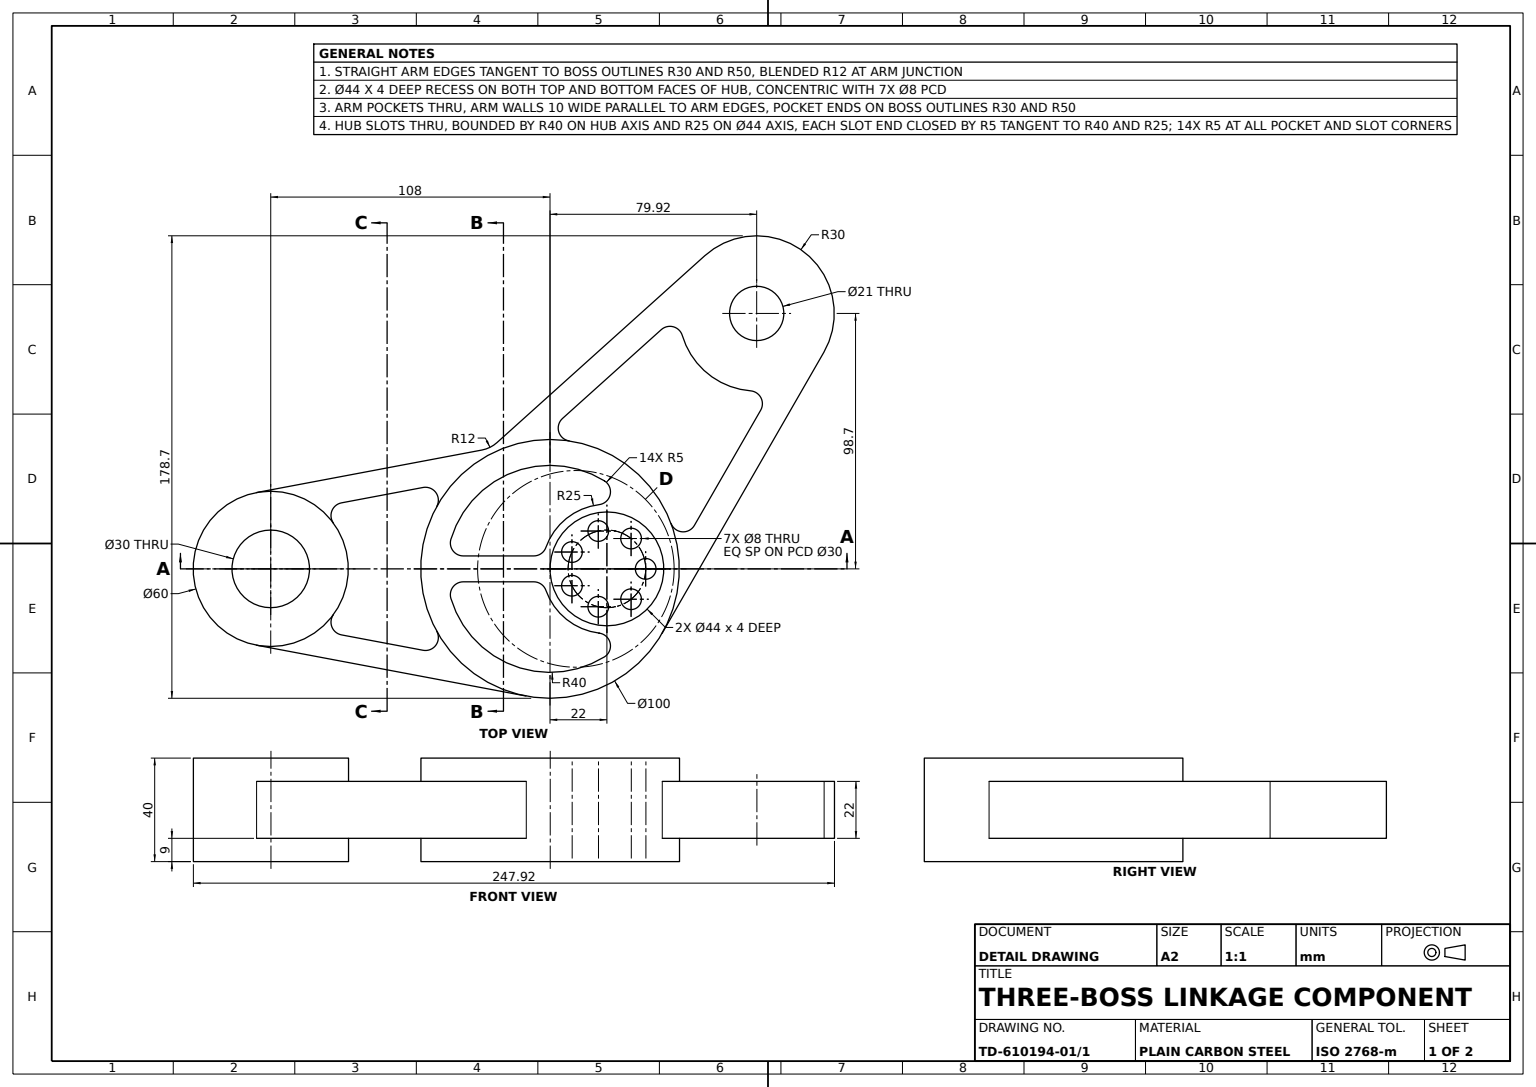
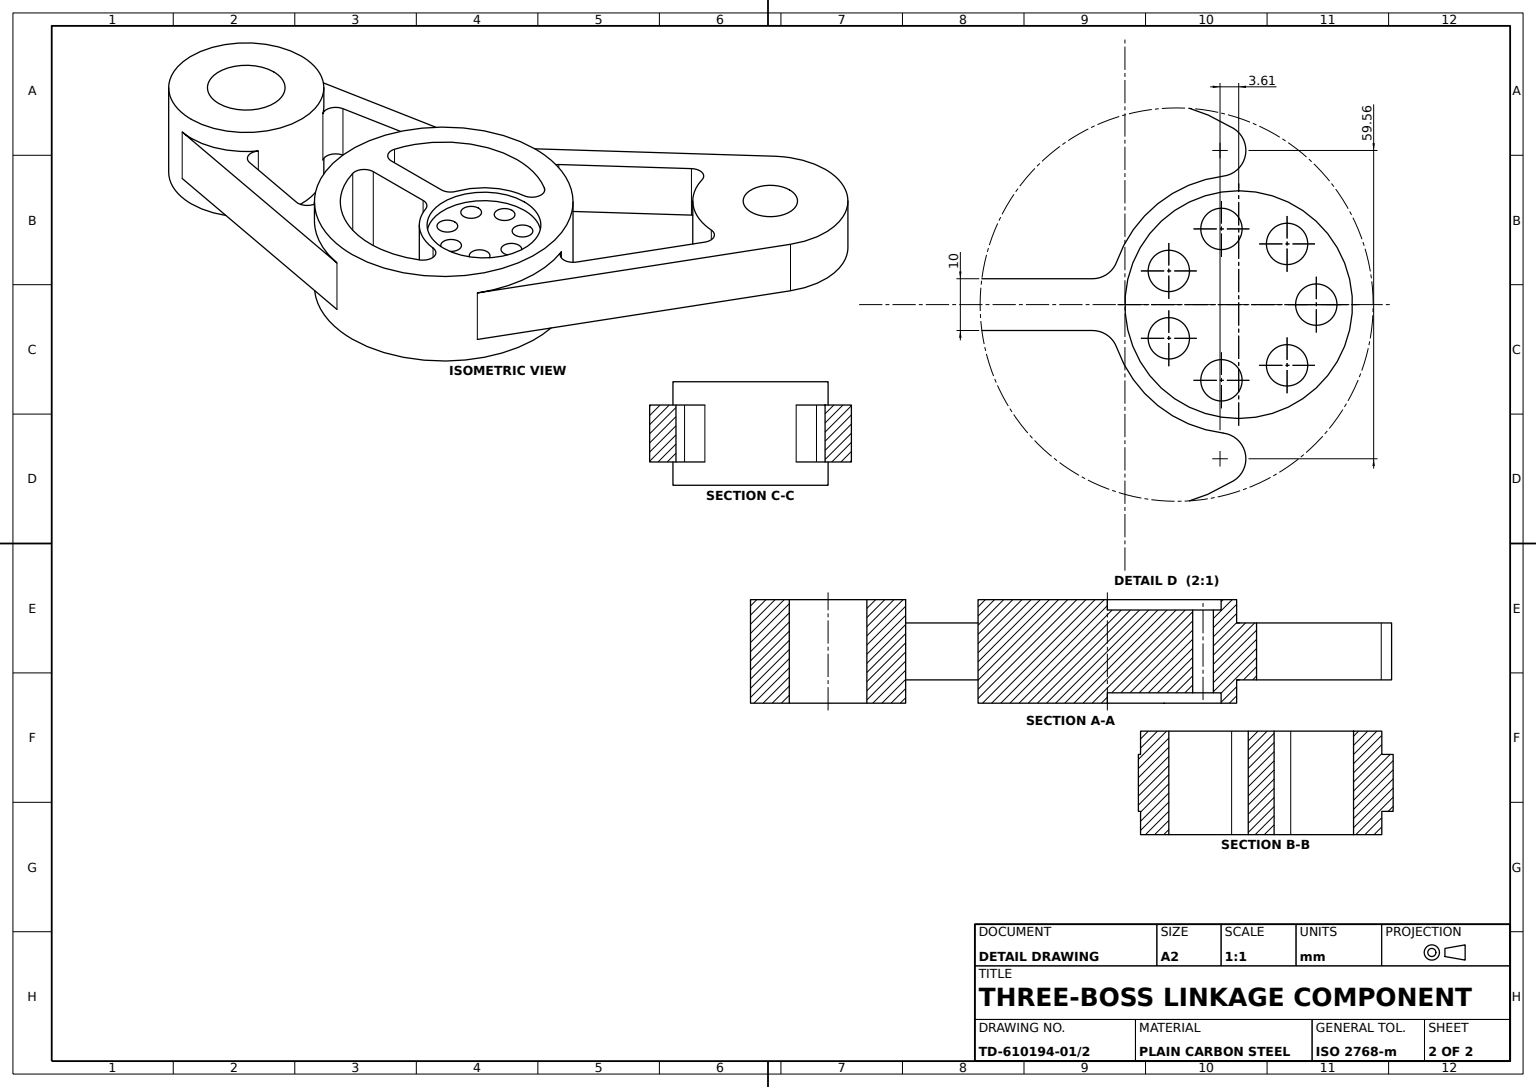
solid
v1 (46.8215331881,11,-17.5426346343)
v2 (46.8215331881,-11,-17.5426346343)
e1 v1 v2 LINE
v3 (55.8364585363,11,-16.8014849975)
e2 v1 v3 CIRCLE(AX(P(51.5036865069,11,-19.2968980978),D(0,1,0),D(0,0,-1)),5)
v4 (55.8364585363,-11,-16.8014849975)
e3 v3 v4 LINE
e4 v2 v4 CIRCLE(AX(P(51.5036865069,-11,-19.2968980978),D(0,1,0),D(0,0,-1)),5)
face CYL(AX(P(51.5036865069,11,-19.2968980978),D(0,-1,0),D(0,0,-1)),5) rev [-e1 e2 e3 -e4]
v5 (22,16,-22)
v6 (22,20,-22)
e5 v5 v6 LINE
v7 (22,16,22)
e6 v7 v5 CIRCLE(AX(P(22,16,0),D(0,1,0),D(0,0,1)),22)
v8 (22,20,22)
e7 v7 v8 LINE
e8 v8 v6 CIRCLE(AX(P(22,20,0),D(0,1,0),D(0,0,1)),22)
face CYL(AX(P(22,16,0),D(0,1,0),D(0,0,1)),22) rev [-e5 -e6 e7 e8]
v9 (-48.1740660132,11,-31.5378854424)
v10 (-43.7946054666,11,-24.1253504021)
e9 v9 v10 CIRCLE(AX(P(-48.1740660132,11,-26.5378854424),D(0,-1,0),D(0,0,1)),5)
v11 (-48.1740660132,-11,-31.5378854424)
e10 v9 v11 LINE
v12 (-43.7946054666,-11,-24.1253504021)
e11 v11 v12 CIRCLE(AX(P(-48.1740660132,-11,-26.5378854424),D(0,-1,0),D(0,0,1)),5)
e12 v10 v12 LINE
face CYL(AX(P(-48.1740660132,11,-26.5378854424),D(0,-1,0),D(0,0,-1)),5) rev [-e9 e10 e11 -e12]
v13 (-80.6278859801,11,25.5101425728)
v14 (-80.6278859801,-11,25.5101425728)
e13 v13 v14 LINE
v15 (-83.7445371893,-11,17.6542494556)
e14 v15 v14 CIRCLE(AX(P(-79.7019600542,-11,20.5966243649),D(0,1,0),D(0,0,-1)),5)
v16 (-83.7445371893,11,17.6542494556)
e15 v16 v15 LINE
e16 v16 v13 CIRCLE(AX(P(-79.7019600542,11,20.5966243649),D(0,1,0),D(0,0,-1)),5)
face CYL(AX(P(-79.7019600542,11,20.5966243649),D(0,-1,0),D(0,0,-1)),5) rev [e13 -e14 -e15 e16]
v17 (18.9886363636,-20,-24.8179710905)
v18 (21.012987013,-20,-34.0360746384)
e17 v17 v18 CIRCLE(AX(P(18.3863636364,-20,-29.7815653086),D(0,1,0),D(0,0,-1)),5)
v19 (18.9886363636,20,-24.8179710905)
e18 v19 v17 LINE
v20 (21.012987013,20,-34.0360746384)
e19 v19 v20 CIRCLE(AX(P(18.3863636364,20,-29.7815653086),D(0,1,0),D(0,0,-1)),5)
e20 v20 v18 LINE
face CYL(AX(P(18.3863636364,11,-29.7815653086),D(0,-1,0),D(0,0,-1)),5) rev [-e17 -e18 e19 e20]
v21 (21.012987013,20,34.0360746384)
v22 (21.012987013,-20,34.0360746384)
e21 v21 v22 LINE
v23 (-38.3325939,-20,11.4285714286)
e22 v23 v22 CIRCLE(AX(P(0,-20,0),D(0,1,0),D(0,0,1)),40)
v24 (-38.3325939,20,11.4285714286)
e23 v24 v23 LINE
e24 v24 v21 CIRCLE(AX(P(0,20,0),D(0,1,0),D(0,0,1)),40)
face CYL(AX(P(0,11,0),D(0,-1,0),D(0,0,-1)),40) rev [e21 -e22 -e23 e24]
v25 (-108,-11,30)
v26 (-108,-20,30)
e25 v25 v26 LINE
v27 (-108,-20,-30)
e26 v26 v27 CIRCLE(AX(P(-108,-20,0),D(0,1,0),D(0,0,1)),30)
v28 (-108,-11,-30)
e27 v28 v27 LINE
v29 (-83.7445371893,-11,-17.6542494556)
e28 v28 v29 CIRCLE(AX(P(-108,-11,0),D(0,-1,0),D(0,0,1)),30)
v30 (-83.7445371893,11,-17.6542494556)
e29 v30 v29 LINE
v31 (-108,11,-30)
e30 v31 v30 CIRCLE(AX(P(-108,11,0),D(0,-1,0),D(0,0,1)),30)
v32 (-108,20,-30)
e31 v32 v31 LINE
v33 (-108,20,30)
e32 v33 v32 CIRCLE(AX(P(-108,20,0),D(0,1,0),D(0,0,1)),30)
v34 (-108,11,30)
e33 v33 v34 LINE
e34 v34 v16 CIRCLE(AX(P(-108,11,0),D(0,1,0),D(0,0,1)),30)
e35 v25 v15 CIRCLE(AX(P(-108,-11,0),D(0,1,0),D(0,0,1)),30)
face CYL(AX(P(-108,20,0),D(0,-1,0),D(0,0,-1)),30) [e25 e26 -e27 e28 -e29 -e30 -e31 -e32 e33 e34 e15 -e35]
v35 (-38.3325939,20,-11.4285714286)
v36 (-38.3325939,-20,-11.4285714286)
e36 v35 v36 LINE
v37 (0,-20,-40)
e37 v37 v36 CIRCLE(AX(P(0,-20,0),D(0,1,0),D(0,0,1)),40)
v38 (0,20,-40)
e38 v38 v37 LINE
e39 v38 v35 CIRCLE(AX(P(0,20,0),D(0,1,0),D(0,0,1)),40)
face CYL(AX(P(0,11,0),D(0,-1,0),D(0,0,-1)),40) rev [e36 -e37 -e38 e39]
v39 (-49.0999919392,-11,-31.4514036503)
e40 v39 v11 CIRCLE(AX(P(-48.1740660132,-11,-26.5378854424),D(0,-1,0),D(0,0,1)),5)
v40 (-49.0999919392,11,-31.4514036503)
e41 v40 v9 CIRCLE(AX(P(-48.1740660132,11,-26.5378854424),D(0,-1,0),D(0,0,1)),5)
e42 v40 v39 LINE
face CYL(AX(P(-48.1740660132,11,-26.5378854424),D(0,-1,0),D(0,0,-1)),5) rev [e40 -e10 -e41 e42]
v41 (81.472399581,11,-61.3130283134)
v42 (81.472399581,-11,-61.3130283134)
e43 v41 v42 LINE
e44 v4 v42 LINE
e45 v3 v41 LINE
face PLANE(AX(P(55.8364585363,11,-16.8014849975),D(-0.8665544059,0,-0.4990826201),D(-0.4990826201,0,0.8665544059))) [e43 -e44 -e3 e45]
v43 (-33.5410196625,-20,5)
e46 v43 v23 CIRCLE(AX(P(-33.5410196625,-20,10),D(0,1,0),D(0,0,1)),5)
v44 (18.9886363636,-20,24.8179710905)
e47 v22 v44 CIRCLE(AX(P(18.3863636364,-20,29.7815653086),D(0,1,0),D(0,0,1)),5)
v45 (-1.5702260396,-20,8.3333333333)
e48 v44 v45 CIRCLE(AX(P(22,-20,0),D(0,-1,0),D(0,0,1)),25)
v46 (-6.2842712475,-20,5)
e49 v45 v46 CIRCLE(AX(P(-6.2842712475,-20,10),D(0,1,0),D(0,0,-1)),5)
e50 v46 v43 LINE
v47 (-33.5410196625,-20,-5)
e51 v36 v47 CIRCLE(AX(P(-33.5410196625,-20,-10),D(0,1,0),D(0,0,-1)),5)
v48 (-6.2842712475,-20,-5)
e52 v47 v48 LINE
v49 (-1.5702260396,-20,-8.3333333333)
e53 v48 v49 CIRCLE(AX(P(-6.2842712475,-20,-10),D(0,1,0),D(0,0,-1)),5)
e54 v49 v17 CIRCLE(AX(P(22,-20,0),D(0,-1,0),D(0,0,1)),25)
e55 v18 v37 CIRCLE(AX(P(0,-20,0),D(0,1,0),D(0,0,1)),40)
v50 (22,-20,22)
v51 (22,-20,-22)
e56 v50 v51 CIRCLE(AX(P(22,-20,0),D(0,1,0),D(0,0,1)),22)
e57 v51 v50 CIRCLE(AX(P(22,-20,0),D(0,1,0),D(0,0,1)),22)
v52 (0,-20,-50)
v53 (0,-20,50)
e58 v52 v53 CIRCLE(AX(P(0,-20,0),D(0,1,0),D(0,0,1)),50)
e59 v53 v52 CIRCLE(AX(P(0,-20,0),D(0,1,0),D(0,0,1)),50)
face PLANE(AX(P(0,-20,0),D(0,1,0),D(0,0,1))) rev [e46 e22 e47 e48 e49 e50] [e51 e52 e53 e54 e17 e55 e37] [e56 e57] [-e58 -e59]
v54 (-108,20,15)
v55 (-108,-20,15)
e60 v54 v55 LINE
v56 (-108,20,-15)
e61 v54 v56 CIRCLE(AX(P(-108,20,0),D(0,1,0),D(0,0,1)),15)
v57 (-108,-20,-15)
e62 v56 v57 LINE
e63 v55 v57 CIRCLE(AX(P(-108,-20,0),D(0,1,0),D(0,0,1)),15)
face CYL(AX(P(-108,20,0),D(0,-1,0),D(0,0,-1)),15) rev [-e60 e61 e62 -e63]
v58 (-33.5410196625,20,-5)
v59 (-6.2842712475,20,-5)
e64 v58 v59 LINE
e65 v59 v48 LINE
e66 v58 v47 LINE
face PLANE(AX(P(-33.5410196625,11,-5),D(0,0,-1),D(-1,0,0))) [e64 e65 -e52 -e66]
v60 (-33.5410196625,20,5)
e67 v60 v43 LINE
v61 (-6.2842712475,20,5)
e68 v61 v46 LINE
e69 v61 v60 LINE
face PLANE(AX(P(-6.2842712475,11,5),D(0,0,1),D(1,0,0))) [e67 -e50 -e68 e69]
v62 (18.6621859907,-16,-10.6239186827)
v63 (18.6621859907,-16,-18.6239186827)
e70 v62 v63 CIRCLE(AX(P(18.6621859907,-16,-14.6239186827),D(0,-1,0),D(0,0,-1)),4)
v64 (18.6621859907,16,-18.6239186827)
e71 v64 v63 LINE
v65 (18.6621859907,16,-10.6239186827)
e72 v64 v65 CIRCLE(AX(P(18.6621859907,16,-14.6239186827),D(0,1,0),D(0,0,1)),4)
e73 v65 v62 LINE
face CYL(AX(P(18.6621859907,20,-14.6239186827),D(0,-1,0),D(0,0,-1)),4) rev [e70 -e71 e72 e73]
e74 v35 v58 CIRCLE(AX(P(-33.5410196625,20,-10),D(0,1,0),D(0,0,-1)),5)
face CYL(AX(P(-33.5410196625,11,-10),D(0,-1,0),D(0,0,-1)),5) rev [e66 -e51 -e36 e74]
v66 (79.9236896633,11,-128.697537105)
v67 (79.9236896633,-11,-128.697537105)
e75 v66 v67 LINE
v68 (105.9203218398,11,-83.7250585032)
e76 v68 v66 CIRCLE(AX(P(79.9236896633,11,-98.697537105),D(0,1,0),D(0,0,1)),30)
v69 (105.9203218398,-11,-83.7250585032)
e77 v68 v69 LINE
e78 v69 v67 CIRCLE(AX(P(79.9236896633,-11,-98.697537105),D(0,1,0),D(0,0,1)),30)
face CYL(AX(P(79.9236896633,11,-98.697537105),D(0,-1,0),D(0,0,-1)),30) [-e75 -e76 e77 e78]
v70 (18.9886363636,20,24.8179710905)
e79 v70 v44 LINE
e80 v21 v70 CIRCLE(AX(P(18.3863636364,20,29.7815653086),D(0,1,0),D(0,0,1)),5)
face CYL(AX(P(18.3863636364,11,29.7815653086),D(0,-1,0),D(0,0,-1)),5) rev [e79 -e47 -e21 e80]
e81 v63 v62 CIRCLE(AX(P(18.6621859907,-16,-14.6239186827),D(0,-1,0),D(0,0,-1)),4)
e82 v65 v64 CIRCLE(AX(P(18.6621859907,16,-14.6239186827),D(0,1,0),D(0,0,1)),4)
face CYL(AX(P(18.6621859907,20,-14.6239186827),D(0,-1,0),D(0,0,-1)),4) rev [e71 e81 -e73 e82]
v71 (37,16,-4)
v72 (37,-16,-4)
e83 v71 v72 LINE
v73 (37,-16,4)
e84 v72 v73 CIRCLE(AX(P(37,-16,0),D(0,-1,0),D(0,0,-1)),4)
v74 (37,16,4)
e85 v74 v73 LINE
e86 v74 v71 CIRCLE(AX(P(37,16,0),D(0,1,0),D(0,0,1)),4)
face CYL(AX(P(37,20,0),D(0,-1,0),D(0,0,-1)),4) rev [e83 e84 -e85 e86]
v75 (59.8733918905,11,-121.0131271537)
v76 (59.8733918905,-11,-121.0131271537)
e87 v75 v76 LINE
v77 (-20.5112949272,-11,-48.7884222029)
e88 v76 v77 LINE
v78 (-20.5112949272,11,-48.7884222029)
e89 v78 v77 LINE
e90 v75 v78 LINE
face PLANE(AX(P(-20.5112949272,11,-48.7884222029),D(0.6683432591,0,0.7438530016),D(0.7438530016,0,-0.6683432591))) rev [e87 e88 -e89 -e90]
e91 v73 v72 CIRCLE(AX(P(37,-16,0),D(0,-1,0),D(0,0,-1)),4)
v79 (18.6621859907,-16,10.6239186827)
v80 (18.6621859907,-16,18.6239186827)
e92 v79 v80 CIRCLE(AX(P(18.6621859907,-16,14.6239186827),D(0,-1,0),D(0,0,-1)),4)
e93 v80 v79 CIRCLE(AX(P(18.6621859907,-16,14.6239186827),D(0,-1,0),D(0,0,-1)),4)
v81 (8.4854669815,-16,-2.5082560868)
v82 (8.4854669815,-16,-10.5082560868)
e94 v81 v82 CIRCLE(AX(P(8.4854669815,-16,-6.5082560868),D(0,-1,0),D(0,0,-1)),4)
e95 v82 v81 CIRCLE(AX(P(8.4854669815,-16,-6.5082560868),D(0,-1,0),D(0,0,-1)),4)
v83 (31.3523470279,-16,15.727472237)
v84 (31.3523470279,-16,7.727472237)
e96 v83 v84 CIRCLE(AX(P(31.3523470279,-16,11.727472237),D(0,-1,0),D(0,0,-1)),4)
e97 v84 v83 CIRCLE(AX(P(31.3523470279,-16,11.727472237),D(0,-1,0),D(0,0,-1)),4)
v85 (22,-16,-22)
v86 (22,-16,22)
e98 v85 v86 CIRCLE(AX(P(22,-16,0),D(0,1,0),D(0,0,1)),22)
e99 v86 v85 CIRCLE(AX(P(22,-16,0),D(0,1,0),D(0,0,1)),22)
v87 (8.4854669815,-16,2.5082560868)
v88 (8.4854669815,-16,10.5082560868)
e100 v87 v88 CIRCLE(AX(P(8.4854669815,-16,6.5082560868),D(0,-1,0),D(0,0,-1)),4)
e101 v88 v87 CIRCLE(AX(P(8.4854669815,-16,6.5082560868),D(0,-1,0),D(0,0,-1)),4)
v89 (31.3523470279,-16,-7.727472237)
v90 (31.3523470279,-16,-15.727472237)
e102 v89 v90 CIRCLE(AX(P(31.3523470279,-16,-11.727472237),D(0,-1,0),D(0,0,-1)),4)
e103 v90 v89 CIRCLE(AX(P(31.3523470279,-16,-11.727472237),D(0,-1,0),D(0,0,-1)),4)
face PLANE(AX(P(22,-16,0),D(0,-1,0),D(0,0,1))) [-e70 -e81] [-e91 -e84] [-e92 -e93] [-e94 -e95] [-e96 -e97] [-e98 -e99] [-e100 -e101] [-e102 -e103]
v91 (-113.5555555556,-11,29.4811092476)
e104 v91 v25 CIRCLE(AX(P(-108,-11,0),D(0,1,0),D(0,0,1)),30)
v92 (-49.0999919392,-11,31.4514036503)
e105 v14 v92 LINE
v93 (-43.7946054666,-11,24.1253504021)
e106 v92 v93 CIRCLE(AX(P(-48.1740660132,-11,26.5378854424),D(0,1,0),D(0,0,1)),5)
v94 (-9.2592592593,-11,49.1351820793)
e107 v94 v93 CIRCLE(AX(P(0,-11,0),D(0,-1,0),D(0,0,1)),50)
e108 v91 v94 LINE
face PLANE(AX(P(-108,-11,0),D(0,1,0),D(0,0,1))) rev [e104 e35 e14 e105 e106 -e107 -e108]
v95 (79.9236896633,11,-88.197537105)
v96 (79.9236896633,-11,-88.197537105)
e109 v95 v96 LINE
v97 (79.9236896633,11,-109.197537105)
e110 v95 v97 CIRCLE(AX(P(79.9236896633,11,-98.697537105),D(0,1,0),D(0,0,1)),10.5)
v98 (79.9236896633,-11,-109.197537105)
e111 v97 v98 LINE
e112 v96 v98 CIRCLE(AX(P(79.9236896633,-11,-98.697537105),D(0,1,0),D(0,0,1)),10.5)
face CYL(AX(P(79.9236896633,11,-98.697537105),D(0,-1,0),D(0,0,-1)),10.5) rev [-e109 e110 e111 -e112]
e113 v66 v75 CIRCLE(AX(P(79.9236896633,11,-98.697537105),D(0,1,0),D(0,0,1)),30)
e114 v67 v76 CIRCLE(AX(P(79.9236896633,-11,-98.697537105),D(0,1,0),D(0,0,1)),30)
face CYL(AX(P(79.9236896633,11,-98.697537105),D(0,-1,0),D(0,0,-1)),30) [-e113 e75 e114 -e87]
v99 (8.4854669815,16,-2.5082560868)
v100 (8.4854669815,16,-10.5082560868)
e115 v99 v100 CIRCLE(AX(P(8.4854669815,16,-6.5082560868),D(0,1,0),D(0,0,1)),4)
e116 v100 v82 LINE
e117 v99 v81 LINE
face CYL(AX(P(8.4854669815,20,-6.5082560868),D(0,-1,0),D(0,0,-1)),4) rev [e115 e116 e95 -e117]
v101 (-26.3091918141,-11,-45.9222145234)
v102 (-113.5555555556,-11,-29.4811092476)
e118 v101 v102 LINE
v103 (-113.5555555556,11,-29.4811092476)
e119 v103 v102 LINE
v104 (-26.3091918141,11,-45.9222145234)
e120 v104 v103 LINE
e121 v104 v101 LINE
face PLANE(AX(P(-26.3091918141,11,-45.9222145234),D(0.1851851852,0,0.9827036416),D(0.9827036416,0,-0.1851851852))) rev [e118 -e119 -e120 e121]
v105 (-113.5555555556,11,29.4811092476)
v106 (-9.2592592593,11,49.1351820793)
e122 v105 v106 LINE
e123 v105 v91 LINE
e124 v106 v94 LINE
face PLANE(AX(P(-113.5555555556,11,29.4811092476),D(0.1851851852,0,-0.9827036416),D(-0.9827036416,0,-0.1851851852))) rev [-e122 e123 e108 -e124]
v107 (-49.0999919392,11,31.4514036503)
v108 (-43.7946054666,11,24.1253504021)
e125 v107 v108 CIRCLE(AX(P(-48.1740660132,11,26.5378854424),D(0,1,0),D(0,0,1)),5)
e126 v108 v93 LINE
e127 v107 v92 LINE
face CYL(AX(P(-48.1740660132,11,26.5378854424),D(0,-1,0),D(0,0,-1)),5) rev [e125 e126 -e106 -e127]
e128 v97 v95 CIRCLE(AX(P(79.9236896633,11,-98.697537105),D(0,1,0),D(0,0,1)),10.5)
e129 v98 v96 CIRCLE(AX(P(79.9236896633,-11,-98.697537105),D(0,1,0),D(0,0,1)),10.5)
face CYL(AX(P(79.9236896633,11,-98.697537105),D(0,-1,0),D(0,0,-1)),10.5) rev [e128 e109 -e129 -e111]
v109 (8.4854669815,16,10.5082560868)
v110 (8.4854669815,16,2.5082560868)
e130 v109 v110 CIRCLE(AX(P(8.4854669815,16,6.5082560868),D(0,1,0),D(0,0,1)),4)
e131 v110 v87 LINE
e132 v109 v88 LINE
face CYL(AX(P(8.4854669815,20,6.5082560868),D(0,-1,0),D(0,0,-1)),4) rev [e130 e131 e100 -e132]
v111 (18.6621859907,16,10.6239186827)
e133 v111 v79 LINE
v112 (18.6621859907,16,18.6239186827)
e134 v112 v80 LINE
e135 v112 v111 CIRCLE(AX(P(18.6621859907,16,14.6239186827),D(0,1,0),D(0,0,1)),4)
face CYL(AX(P(18.6621859907,20,14.6239186827),D(0,-1,0),D(0,0,-1)),4) rev [e133 e92 -e134 e135]
e136 v5 v7 CIRCLE(AX(P(22,16,0),D(0,1,0),D(0,0,1)),22)
v113 (31.3523470279,16,-7.727472237)
v114 (31.3523470279,16,-15.727472237)
e137 v113 v114 CIRCLE(AX(P(31.3523470279,16,-11.727472237),D(0,1,0),D(0,0,1)),4)
e138 v114 v113 CIRCLE(AX(P(31.3523470279,16,-11.727472237),D(0,1,0),D(0,0,1)),4)
e139 v111 v112 CIRCLE(AX(P(18.6621859907,16,14.6239186827),D(0,1,0),D(0,0,1)),4)
v115 (31.3523470279,16,7.727472237)
v116 (31.3523470279,16,15.727472237)
e140 v115 v116 CIRCLE(AX(P(31.3523470279,16,11.727472237),D(0,1,0),D(0,0,1)),4)
e141 v116 v115 CIRCLE(AX(P(31.3523470279,16,11.727472237),D(0,1,0),D(0,0,1)),4)
e142 v71 v74 CIRCLE(AX(P(37,16,0),D(0,1,0),D(0,0,1)),4)
e143 v110 v109 CIRCLE(AX(P(8.4854669815,16,6.5082560868),D(0,1,0),D(0,0,1)),4)
e144 v100 v99 CIRCLE(AX(P(8.4854669815,16,-6.5082560868),D(0,1,0),D(0,0,1)),4)
face PLANE(AX(P(22,16,0),D(0,1,0),D(0,0,1))) [e6 e136] [-e137 -e138] [-e135 -e139] [-e140 -e141] [-e86 -e142] [-e130 -e143] [-e82 -e72] [-e144 -e115]
e145 v13 v107 LINE
face PLANE(AX(P(-80.6278859801,11,25.5101425728),D(0.1851851852,0,-0.9827036416),D(-0.9827036416,0,-0.1851851852))) [e127 -e105 -e13 e145]
e146 v114 v90 LINE
e147 v113 v89 LINE
face CYL(AX(P(31.3523470279,20,-11.727472237),D(0,-1,0),D(0,0,-1)),4) rev [e137 e146 e103 -e147]
e148 v116 v83 LINE
e149 v115 v84 LINE
face CYL(AX(P(31.3523470279,20,11.727472237),D(0,-1,0),D(0,0,-1)),4) rev [e140 e148 e96 -e149]
e150 v60 v24 CIRCLE(AX(P(-33.5410196625,20,10),D(0,1,0),D(0,0,1)),5)
face CYL(AX(P(-33.5410196625,11,10),D(0,-1,0),D(0,0,-1)),5) rev [e150 e23 -e46 -e67]
v117 (-1.5702260396,20,8.3333333333)
e151 v117 v45 LINE
e152 v117 v61 CIRCLE(AX(P(-6.2842712475,20,10),D(0,1,0),D(0,0,-1)),5)
face CYL(AX(P(-6.2842712475,11,10),D(0,-1,0),D(0,0,-1)),5) rev [-e151 e152 e68 -e49]
e153 v57 v55 CIRCLE(AX(P(-108,-20,0),D(0,1,0),D(0,0,1)),15)
e154 v27 v26 CIRCLE(AX(P(-108,-20,0),D(0,1,0),D(0,0,1)),30)
face PLANE(AX(P(-108,-20,0),D(0,1,0),D(0,0,1))) rev [e153 e63] [-e154 -e26]
e155 v70 v117 CIRCLE(AX(P(22,20,0),D(0,-1,0),D(0,0,1)),25)
face CYL(AX(P(22,11,0),D(0,-1,0),D(0,0,-1)),25) [-e79 e155 e151 -e48]
face CYL(AX(P(31.3523470279,20,11.727472237),D(0,-1,0),D(0,0,-1)),4) rev [e141 e149 e97 -e148]
face CYL(AX(P(37,20,0),D(0,-1,0),D(0,0,-1)),4) rev [e142 e85 e91 -e83]
v118 (-1.5702260396,20,-8.3333333333)
e156 v118 v49 LINE
e157 v59 v118 CIRCLE(AX(P(-6.2842712475,20,-10),D(0,1,0),D(0,0,-1)),5)
face CYL(AX(P(-6.2842712475,11,-10),D(0,-1,0),D(0,0,-1)),5) rev [e156 -e53 -e65 e157]
e158 v56 v54 CIRCLE(AX(P(-108,20,0),D(0,1,0),D(0,0,1)),15)
face CYL(AX(P(-108,20,0),D(0,-1,0),D(0,0,-1)),15) rev [-e62 e158 e60 -e153]
e159 v6 v8 CIRCLE(AX(P(22,20,0),D(0,1,0),D(0,0,1)),22)
face CYL(AX(P(22,16,0),D(0,1,0),D(0,0,1)),22) rev [-e136 e5 e159 -e7]
v119 (0,20,-50)
v120 (0,20,50)
e160 v119 v120 CIRCLE(AX(P(0,20,0),D(0,1,0),D(0,0,1)),50)
e161 v120 v119 CIRCLE(AX(P(0,20,0),D(0,1,0),D(0,0,1)),50)
e162 v118 v19 CIRCLE(AX(P(22,20,0),D(0,-1,0),D(0,0,1)),25)
e163 v20 v38 CIRCLE(AX(P(0,20,0),D(0,1,0),D(0,0,1)),40)
face PLANE(AX(P(0,20,0),D(0,1,0),D(0,0,1))) [e160 e161] [-e19 -e162 -e157 -e64 -e74 -e39 -e163] [-e8 -e159] [-e152 -e155 -e80 -e24 -e150 -e69]
face CYL(AX(P(31.3523470279,20,-11.727472237),D(0,-1,0),D(0,0,-1)),4) rev [-e146 e138 e147 e102]
v121 (-80.6278859801,-11,-25.5101425728)
e164 v29 v121 CIRCLE(AX(P(-79.7019600542,-11,-20.5966243649),D(0,-1,0),D(0,0,1)),5)
v122 (-80.6278859801,11,-25.5101425728)
e165 v122 v121 LINE
e166 v30 v122 CIRCLE(AX(P(-79.7019600542,11,-20.5966243649),D(0,-1,0),D(0,0,1)),5)
face CYL(AX(P(-79.7019600542,11,-20.5966243649),D(0,-1,0),D(0,0,-1)),5) rev [e164 -e165 -e166 e29]
v123 (77.5373507104,11,-68.7925979411)
v124 (77.5373507104,-11,-68.7925979411)
e167 v123 v124 LINE
e168 v42 v124 CIRCLE(AX(P(77.1396275515,-11,-63.8084414137),D(0,1,0),D(0,0,1)),5)
e169 v41 v123 CIRCLE(AX(P(77.1396275515,11,-63.8084414137),D(0,1,0),D(0,0,1)),5)
face CYL(AX(P(77.1396275515,11,-63.8084414137),D(0,-1,0),D(0,0,-1)),5) rev [e167 -e168 -e43 e169]
v125 (43.0341271866,-11,-92.4397275619)
v126 (4.8252797355,-11,-58.1095231049)
e170 v125 v126 LINE
v127 (43.0341271866,11,-92.4397275619)
e171 v127 v125 LINE
v128 (4.8252797355,11,-58.1095231049)
e172 v127 v128 LINE
e173 v128 v126 LINE
face PLANE(AX(P(4.8252797355,11,-58.1095231049),D(0.6683432591,0,0.7438530016),D(0.7438530016,0,-0.6683432591))) [-e170 -e171 e172 e173]
face CYL(AX(P(8.4854669815,20,6.5082560868),D(0,-1,0),D(0,0,-1)),4) rev [e143 e132 e101 -e131]
v129 (51.1683929366,11,-90.1457589183)
v130 (51.1683929366,-11,-90.1457589183)
e174 v129 v130 LINE
v131 (46.3758434821,11,-93.7204625538)
e175 v129 v131 CIRCLE(AX(P(46.3758434821,11,-88.7204625538),D(0,1,0),D(0,0,-1)),5)
v132 (46.3758434821,-11,-93.7204625538)
e176 v131 v132 LINE
e177 v130 v132 CIRCLE(AX(P(46.3758434821,-11,-88.7204625538),D(0,1,0),D(0,0,-1)),5)
face CYL(AX(P(46.3758434821,11,-88.7204625538),D(0,-1,0),D(0,0,-1)),5) rev [-e174 e175 e176 -e177]
e178 v131 v127 CIRCLE(AX(P(46.3758434821,11,-88.7204625538),D(0,1,0),D(0,0,-1)),5)
e179 v132 v125 CIRCLE(AX(P(46.3758434821,-11,-88.7204625538),D(0,1,0),D(0,0,-1)),5)
face CYL(AX(P(46.3758434821,11,-88.7204625538),D(0,-1,0),D(0,0,-1)),5) rev [e178 e171 -e179 -e176]
e180 v86 v50 LINE
e181 v85 v51 LINE
face CYL(AX(P(22,-16,0),D(0,-1,0),D(0,0,-1)),22) rev [e98 e180 -e57 -e181]
e182 v32 v33 CIRCLE(AX(P(-108,20,0),D(0,1,0),D(0,0,1)),30)
face PLANE(AX(P(-108,20,0),D(0,1,0),D(0,0,1))) [e182 e32] [-e61 -e158]
face CYL(AX(P(8.4854669815,20,-6.5082560868),D(0,-1,0),D(0,0,-1)),4) rev [e144 e117 e94 -e116]
v133 (7.4245418463,11,-49.4456891789)
e183 v128 v133 CIRCLE(AX(P(8.1669960309,11,-54.3902580967),D(0,1,0),D(0,0,1)),5)
v134 (7.4245418463,-11,-49.4456891789)
e184 v133 v134 LINE
e185 v126 v134 CIRCLE(AX(P(8.1669960309,-11,-54.3902580967),D(0,1,0),D(0,0,1)),5)
face CYL(AX(P(8.1669960309,11,-54.3902580967),D(0,-1,0),D(0,0,-1)),5) rev [e183 e184 -e185 -e173]
e186 v129 v123 CIRCLE(AX(P(79.9236896633,11,-98.697537105),D(0,1,0),D(0,0,1)),30)
e187 v130 v124 CIRCLE(AX(P(79.9236896633,-11,-98.697537105),D(0,1,0),D(0,0,1)),30)
face CYL(AX(P(79.9236896633,11,-98.697537105),D(0,-1,0),D(0,0,-1)),30) [-e186 e174 e187 -e167]
v135 (43.3277202941,-11,24.9541310031)
e188 v135 v69 LINE
v136 (43.3277202941,11,24.9541310031)
e189 v136 v68 LINE
e190 v136 v135 LINE
face PLANE(AX(P(43.3277202941,11,24.9541310031),D(-0.8665544059,0,-0.4990826201),D(-0.4990826201,0,0.8665544059))) rev [e188 -e77 -e189 e190]
face CYL(AX(P(22,-16,0),D(0,-1,0),D(0,0,-1)),22) rev [e99 e181 -e56 -e180]
e191 v1 v136 CIRCLE(AX(P(0,11,0),D(0,-1,0),D(0,0,1)),50)
e192 v2 v135 CIRCLE(AX(P(0,-11,0),D(0,-1,0),D(0,0,1)),50)
v137 (0,-11,-50)
e193 v137 v52 LINE
e194 v137 v134 CIRCLE(AX(P(0,-11,0),D(0,-1,0),D(0,0,1)),50)
v138 (0,11,-50)
e195 v138 v133 CIRCLE(AX(P(0,11,0),D(0,-1,0),D(0,0,1)),50)
e196 v119 v138 LINE
e197 v120 v53 LINE
face CYL(AX(P(0,11,0),D(0,-1,0),D(0,0,-1)),50) [-e190 -e191 e1 e192] [-e193 e194 -e184 -e195 -e196 -e161 e197 e59]
e198 v10 v138 CIRCLE(AX(P(0,11,0),D(0,-1,0),D(0,0,1)),50)
e199 v12 v137 CIRCLE(AX(P(0,-11,0),D(0,-1,0),D(0,0,1)),50)
e200 v106 v108 CIRCLE(AX(P(0,11,0),D(0,-1,0),D(0,0,1)),50)
face CYL(AX(P(0,11,0),D(0,-1,0),D(0,0,-1)),50) [e58 -e197 -e160 e196 -e198 e12 e199 e193] [-e200 e124 e107 -e126]
e201 v102 v28 CIRCLE(AX(P(-108,-11,0),D(0,-1,0),D(0,0,1)),30)
e202 v105 v34 CIRCLE(AX(P(-108,11,0),D(0,1,0),D(0,0,1)),30)
e203 v103 v31 CIRCLE(AX(P(-108,11,0),D(0,-1,0),D(0,0,1)),30)
face CYL(AX(P(-108,20,0),D(0,-1,0),D(0,0,-1)),30) [e119 e201 e27 e154 -e25 -e104 -e123 e202 -e33 -e182 e31 -e203]
e204 v78 v104 CIRCLE(AX(P(-28.5314140364,11,-57.7146582224),D(0,-1,0),D(0,0,-1)),12)
e205 v122 v40 LINE
face PLANE(AX(P(79.9236896633,11,-98.697537105),D(0,1,0),D(0,0,1))) [-e110 -e128] [e41 e9 e198 e195 -e183 -e172 -e178 -e175 e186 -e169 -e45 -e2 e191 e189 e76 e113 e90 e204 e120 e203 e30 e166 e205]
face CYL(AX(P(0,11,0),D(0,-1,0),D(0,0,-1)),40) rev [-e20 e163 e38 -e55]
e206 v77 v101 CIRCLE(AX(P(-28.5314140364,-11,-57.7146582224),D(0,-1,0),D(0,0,-1)),12)
e207 v121 v39 LINE
face PLANE(AX(P(79.9236896633,-11,-98.697537105),D(0,1,0),D(0,0,1))) rev [e112 e129] [-e201 -e118 -e206 -e88 -e114 -e78 -e188 -e192 e4 e44 e168 -e187 e177 e179 e170 e185 -e194 -e199 -e11 -e40 -e207 -e164 -e28]
face PLANE(AX(P(-108,11,0),D(0,1,0),D(0,0,1))) [-e145 -e16 -e34 -e202 e122 e200 -e125]
face CYL(AX(P(22,11,0),D(0,-1,0),D(0,0,-1)),25) [e162 e18 -e54 -e156]
face PLANE(AX(P(-49.0999919392,11,-31.4514036503),D(-0.1851851852,0,-0.9827036416),D(-0.9827036416,0,0.1851851852))) rev [-e42 -e205 e165 e207]
face CYL(AX(P(18.6621859907,20,14.6239186827),D(0,-1,0),D(0,0,-1)),4) rev [-e133 e139 e134 e93]
face CYL(AX(P(-28.5314140364,11,-57.7146582224),D(0,-1,0),D(0,0,-1)),12) rev [e206 -e121 -e204 e89]
